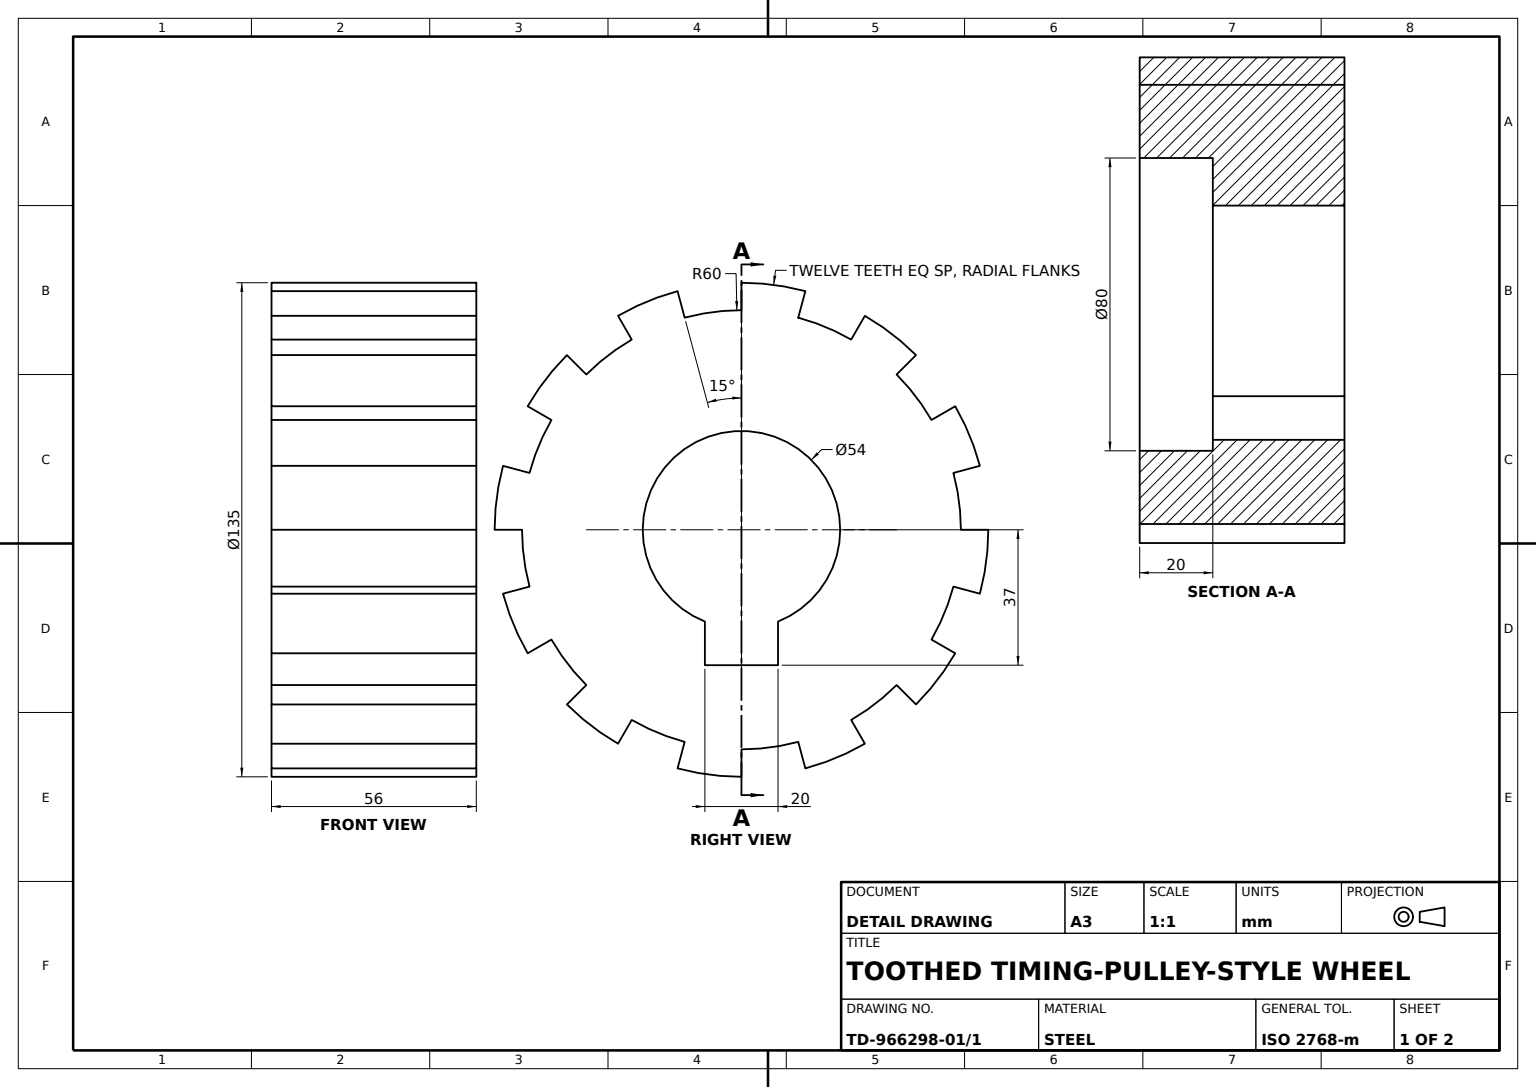
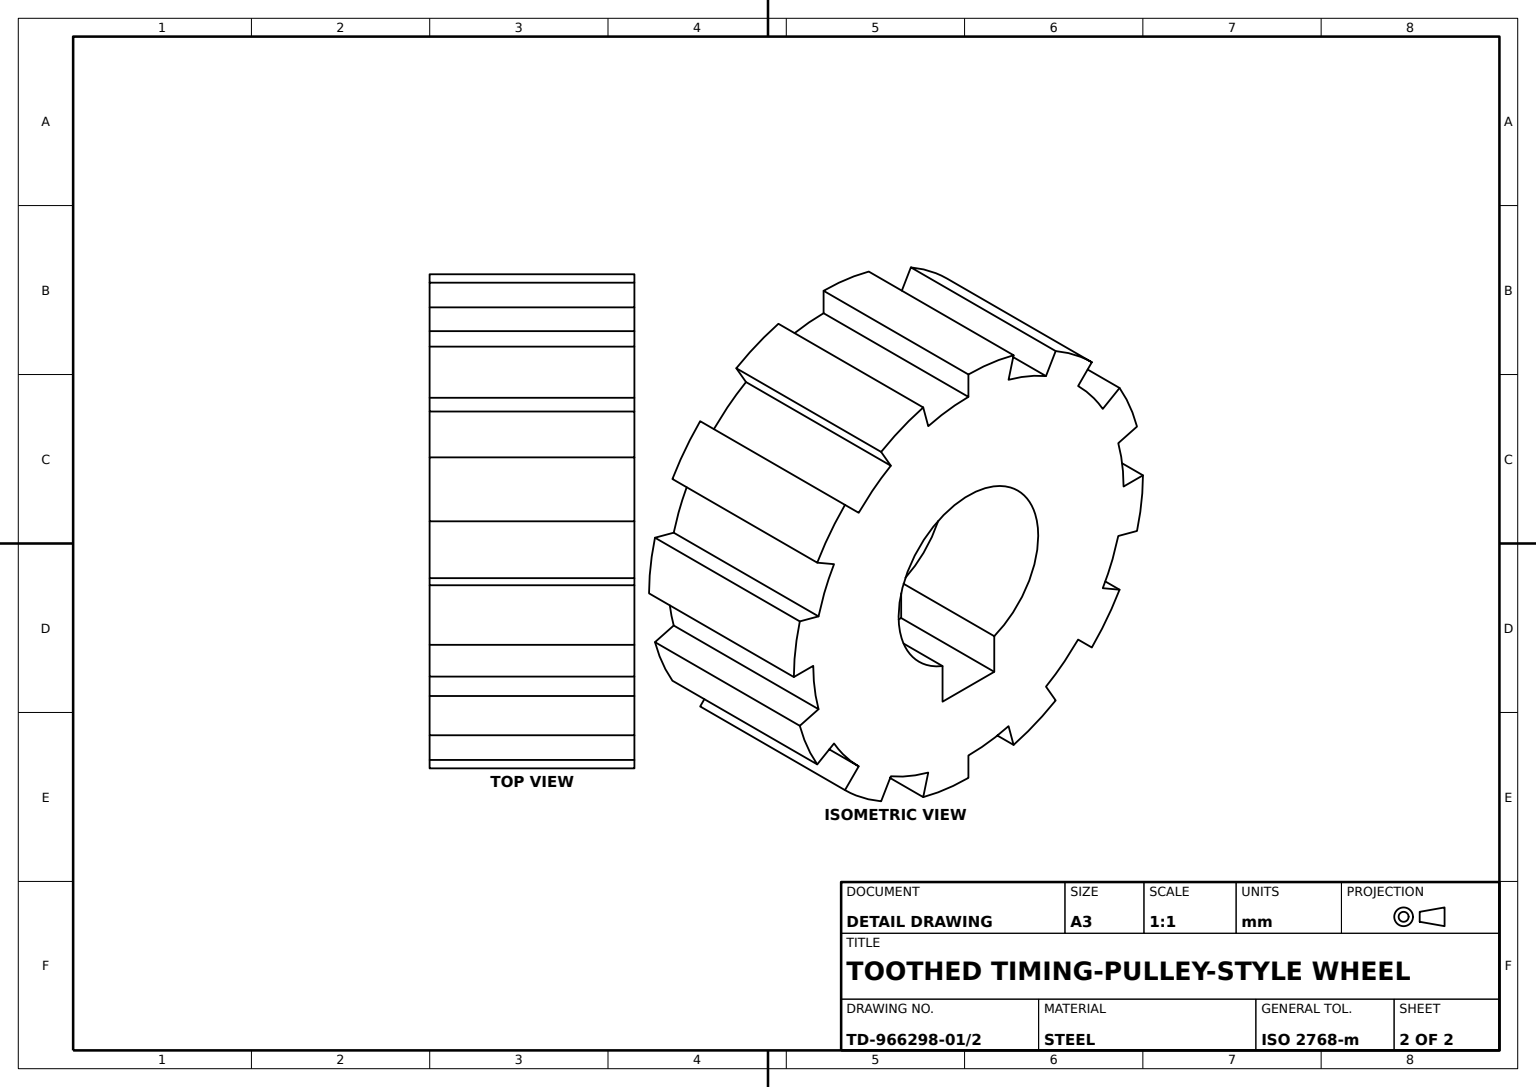
solid
v1 (10,-37,-56)
v2 (10,-37,-20)
e1 v1 v2 LINE
v3 (10,-25.079872,-20)
e2 v2 v3 LINE
v4 (10,-25.079872,-56)
e3 v4 v3 LINE
e4 v1 v4 LINE
face PLANE(AX(P(10,-37,-56),D(1,0,0),D(0,0,-1))) rev [e1 e2 -e3 -e4]
v5 (-47.729708,-47.729708,-56)
v6 (-47.729708,-47.729708,0)
e5 v5 v6 LINE
v7 (-42.426407,-42.426407,-56)
e6 v7 v5 LINE
v8 (-42.426407,-42.426407,0)
e7 v7 v8 LINE
e8 v8 v6 LINE
face PLANE(AX(P(0,0,-56),D(-0.707106781,0.707106781,0),D(-0.707106781,-0.707106781,0))) rev [-e5 -e6 e7 e8]
v9 (57.95555,-15.529143,0)
v10 (60,0,0)
e9 v9 v10 CIRCLE(AX(P(0,0,0),D(0,0,1),D(1,0,0)),60)
v11 (57.95555,-15.529143,-56)
e10 v11 v9 LINE
v12 (60,0,-56)
e11 v11 v12 CIRCLE(AX(P(0,0,-56),D(0,0,1),D(1,0,0)),60)
e12 v12 v10 LINE
face CYL(AX(P(0,0,-56),D(0,0,1),D(1,0,0)),60) [-e9 -e10 e11 e12]
v13 (65.199993,-17.470286,-56)
v14 (65.199993,-17.470286,0)
e13 v13 v14 LINE
e14 v11 v13 LINE
e15 v9 v14 LINE
face PLANE(AX(P(0,0,-56),D(-0.258819045,-0.965925826,0),D(0.965925826,-0.258819045,0))) rev [-e13 -e14 e10 e15]
v15 (-57.95555,15.529143,-56)
v16 (-57.95555,15.529143,0)
e16 v15 v16 LINE
v17 (-60,0,-56)
e17 v15 v17 CIRCLE(AX(P(0,0,-56),D(0,0,1),D(1,0,0)),60)
v18 (-60,0,0)
e18 v17 v18 LINE
e19 v16 v18 CIRCLE(AX(P(0,0,0),D(0,0,1),D(1,0,0)),60)
face CYL(AX(P(0,0,-56),D(0,0,1),D(1,0,0)),60) [-e16 e17 e18 -e19]
v19 (17.470286,65.199993,-56)
v20 (17.470286,65.199993,0)
e20 v19 v20 LINE
v21 (15.529143,57.95555,-56)
e21 v21 v19 LINE
v22 (15.529143,57.95555,0)
e22 v21 v22 LINE
e23 v22 v20 LINE
face PLANE(AX(P(0,0,-56),D(0.965925826,-0.258819045,0),D(0.258819045,0.965925826,0))) rev [-e20 -e21 e22 e23]
v23 (58.456715,-33.75,0)
e24 v23 v14 CIRCLE(AX(P(0,0,0),D(0,0,1),D(1,0,0)),67.5)
v24 (58.456715,-33.75,-56)
e25 v24 v23 LINE
e26 v24 v13 CIRCLE(AX(P(0,0,-56),D(0,0,1),D(1,0,0)),67.5)
face CYL(AX(P(0,0,-56),D(0,0,1),D(1,0,0)),67.5) [-e24 -e25 e26 e13]
v25 (42.426407,-42.426407,-56)
v26 (47.729708,-47.729708,-56)
e27 v25 v26 LINE
v27 (42.426407,-42.426407,0)
e28 v25 v27 LINE
v28 (47.729708,-47.729708,0)
e29 v27 v28 LINE
e30 v26 v28 LINE
face PLANE(AX(P(0,0,-56),D(-0.707106781,-0.707106781,0),D(0.707106781,-0.707106781,0))) rev [-e27 e28 e29 -e30]
v29 (67.5,0,-56)
v30 (67.5,0,0)
e31 v29 v30 LINE
e32 v10 v30 LINE
e33 v12 v29 LINE
face PLANE(AX(P(0,0,-56),D(0,-1,0),D(1,0,0))) [e31 -e32 -e12 e33]
v31 (40,0,-20)
v32 (40,0,0)
e34 v31 v32 LINE
v33 (-40,0,-20)
e35 v33 v31 CIRCLE(AX(P(0,0,-20),D(0,0,1),D(1,0,0)),40)
v34 (-40,0,0)
e36 v33 v34 LINE
e37 v34 v32 CIRCLE(AX(P(0,0,0),D(0,0,1),D(1,0,0)),40)
face CYL(AX(P(0,0,-20),D(0,0,1),D(1,0,0)),40) rev [-e34 -e35 e36 e37]
v35 (-33.75,-58.456715,-56)
v36 (-17.470286,-65.199993,-56)
e38 v35 v36 CIRCLE(AX(P(0,0,-56),D(0,0,1),D(1,0,0)),67.5)
v37 (-17.470286,-65.199993,0)
e39 v36 v37 LINE
v38 (-33.75,-58.456715,0)
e40 v38 v37 CIRCLE(AX(P(0,0,0),D(0,0,1),D(1,0,0)),67.5)
e41 v35 v38 LINE
face CYL(AX(P(0,0,-56),D(0,0,1),D(1,0,0)),67.5) [e38 e39 -e40 -e41]
v39 (0,-67.5,0)
v40 (17.470286,-65.199993,0)
e42 v39 v40 CIRCLE(AX(P(0,0,0),D(0,0,1),D(1,0,0)),67.5)
v41 (0,-67.5,-56)
e43 v41 v39 LINE
v42 (17.470286,-65.199993,-56)
e44 v41 v42 CIRCLE(AX(P(0,0,-56),D(0,0,1),D(1,0,0)),67.5)
e45 v42 v40 LINE
face CYL(AX(P(0,0,-56),D(0,0,1),D(1,0,0)),67.5) [-e42 -e43 e44 e45]
v43 (0,-60,-56)
v44 (0,-60,0)
e46 v43 v44 LINE
v45 (-15.529143,-57.95555,0)
e47 v45 v44 CIRCLE(AX(P(0,0,0),D(0,0,1),D(1,0,0)),60)
v46 (-15.529143,-57.95555,-56)
e48 v46 v45 LINE
e49 v46 v43 CIRCLE(AX(P(0,0,-56),D(0,0,1),D(1,0,0)),60)
face CYL(AX(P(0,0,-56),D(0,0,1),D(1,0,0)),60) [e46 -e47 -e48 e49]
e50 v44 v39 LINE
e51 v43 v41 LINE
face PLANE(AX(P(0,0,-56),D(-1,0,0),D(0,-1,0))) [-e50 -e46 e51 e43]
v47 (-58.456715,33.75,-56)
v48 (-58.456715,33.75,0)
e52 v47 v48 LINE
v49 (-65.199993,17.470286,-56)
e53 v47 v49 CIRCLE(AX(P(0,0,-56),D(0,0,1),D(1,0,0)),67.5)
v50 (-65.199993,17.470286,0)
e54 v49 v50 LINE
e55 v48 v50 CIRCLE(AX(P(0,0,0),D(0,0,1),D(1,0,0)),67.5)
face CYL(AX(P(0,0,-56),D(0,0,1),D(1,0,0)),67.5) [-e52 e53 e54 -e55]
v51 (-30,-51.961524,-56)
e56 v51 v35 LINE
v52 (-30,-51.961524,0)
e57 v52 v38 LINE
e58 v51 v52 LINE
face PLANE(AX(P(0,0,-56),D(-0.866025404,0.5,0),D(-0.5,-0.866025404,0))) [e56 e41 -e57 -e58]
e59 v16 v50 LINE
e60 v15 v49 LINE
face PLANE(AX(P(0,0,-56),D(0.258819045,0.965925826,0),D(-0.965925826,0.258819045,0))) rev [e59 -e54 -e60 e16]
v53 (-57.95555,-15.529143,-56)
v54 (-57.95555,-15.529143,0)
e61 v53 v54 LINE
v55 (-51.961524,-30,-56)
e62 v53 v55 CIRCLE(AX(P(0,0,-56),D(0,0,1),D(1,0,0)),60)
v56 (-51.961524,-30,0)
e63 v55 v56 LINE
e64 v54 v56 CIRCLE(AX(P(0,0,0),D(0,0,1),D(1,0,0)),60)
face CYL(AX(P(0,0,-56),D(0,0,1),D(1,0,0)),60) [-e61 e62 e63 -e64]
v57 (-67.5,0,-56)
v58 (-65.199993,-17.470286,-56)
e65 v57 v58 CIRCLE(AX(P(0,0,-56),D(0,0,1),D(1,0,0)),67.5)
v59 (-65.199993,-17.470286,0)
e66 v58 v59 LINE
v60 (-67.5,0,0)
e67 v60 v59 CIRCLE(AX(P(0,0,0),D(0,0,1),D(1,0,0)),67.5)
e68 v57 v60 LINE
face CYL(AX(P(0,0,-56),D(0,0,1),D(1,0,0)),67.5) [e65 e66 -e67 -e68]
v61 (-33.75,58.456715,-56)
v62 (-33.75,58.456715,0)
e69 v61 v62 LINE
v63 (-30,51.961524,0)
e70 v63 v62 LINE
v64 (-30,51.961524,-56)
e71 v64 v63 LINE
e72 v64 v61 LINE
face PLANE(AX(P(0,0,-56),D(0.866025404,0.5,0),D(-0.5,0.866025404,0))) [e69 -e70 -e71 e72]
e73 v31 v33 CIRCLE(AX(P(0,0,-20),D(0,0,1),D(1,0,0)),40)
v65 (27,0,-20)
v66 (-27,0,-20)
e74 v65 v66 CIRCLE(AX(P(0,0,-20),D(0,0,1),D(1,0,0)),27)
e75 v3 v65 CIRCLE(AX(P(0,0,-20),D(0,0,1),D(1,0,0)),27)
v67 (-10,-37,-20)
e76 v67 v2 LINE
v68 (-10,-25.079872,-20)
e77 v68 v67 LINE
e78 v66 v68 CIRCLE(AX(P(0,0,-20),D(0,0,1),D(1,0,0)),27)
face PLANE(AX(P(0,0,-20),D(0,0,1),D(1,0,0))) [e35 e73] [-e74 -e75 -e2 -e76 -e77 -e78]
v69 (-15.529143,57.95555,0)
v70 (-17.470286,65.199993,0)
e79 v69 v70 LINE
v71 (-17.470286,65.199993,-56)
e80 v71 v70 LINE
v72 (-15.529143,57.95555,-56)
e81 v72 v71 LINE
e82 v72 v69 LINE
face PLANE(AX(P(0,0,-56),D(0.965925826,0.258819045,0),D(-0.258819045,0.965925826,0))) rev [e79 -e80 -e81 e82]
v73 (65.199993,17.470286,-56)
e83 v29 v73 CIRCLE(AX(P(0,0,-56),D(0,0,1),D(1,0,0)),67.5)
v74 (65.199993,17.470286,0)
e84 v73 v74 LINE
e85 v30 v74 CIRCLE(AX(P(0,0,0),D(0,0,1),D(1,0,0)),67.5)
face CYL(AX(P(0,0,-56),D(0,0,1),D(1,0,0)),67.5) [e83 e84 -e85 -e31]
v75 (30,-51.961524,-56)
v76 (30,-51.961524,0)
e86 v75 v76 LINE
v77 (15.529143,-57.95555,0)
e87 v77 v76 CIRCLE(AX(P(0,0,0),D(0,0,1),D(1,0,0)),60)
v78 (15.529143,-57.95555,-56)
e88 v78 v77 LINE
e89 v78 v75 CIRCLE(AX(P(0,0,-56),D(0,0,1),D(1,0,0)),60)
face CYL(AX(P(0,0,-56),D(0,0,1),D(1,0,0)),60) [e86 -e87 -e88 e89]
v79 (33.75,-58.456715,-56)
e90 v79 v26 CIRCLE(AX(P(0,0,-56),D(0,0,1),D(1,0,0)),67.5)
v80 (33.75,-58.456715,0)
e91 v80 v28 CIRCLE(AX(P(0,0,0),D(0,0,1),D(1,0,0)),67.5)
e92 v79 v80 LINE
face CYL(AX(P(0,0,-56),D(0,0,1),D(1,0,0)),67.5) [e90 e30 -e91 -e92]
v81 (33.75,58.456715,0)
e93 v81 v20 CIRCLE(AX(P(0,0,0),D(0,0,1),D(1,0,0)),67.5)
v82 (33.75,58.456715,-56)
e94 v82 v81 LINE
e95 v82 v19 CIRCLE(AX(P(0,0,-56),D(0,0,1),D(1,0,0)),67.5)
face CYL(AX(P(0,0,-56),D(0,0,1),D(1,0,0)),67.5) [e20 -e93 -e94 e95]
v83 (-58.456715,-33.75,-56)
v84 (-58.456715,-33.75,0)
e96 v83 v84 LINE
e97 v83 v5 CIRCLE(AX(P(0,0,-56),D(0,0,1),D(1,0,0)),67.5)
e98 v84 v6 CIRCLE(AX(P(0,0,0),D(0,0,1),D(1,0,0)),67.5)
face CYL(AX(P(0,0,-56),D(0,0,1),D(1,0,0)),67.5) [-e96 e97 e5 -e98]
v85 (51.961524,30,-56)
v86 (51.961524,30,0)
e99 v85 v86 LINE
v87 (57.95555,15.529143,0)
e100 v87 v86 CIRCLE(AX(P(0,0,0),D(0,0,1),D(1,0,0)),60)
v88 (57.95555,15.529143,-56)
e101 v88 v87 LINE
e102 v88 v85 CIRCLE(AX(P(0,0,-56),D(0,0,1),D(1,0,0)),60)
face CYL(AX(P(0,0,-56),D(0,0,1),D(1,0,0)),60) [e99 -e100 -e101 e102]
v89 (58.456715,33.75,-56)
v90 (58.456715,33.75,0)
e103 v89 v90 LINE
e104 v86 v90 LINE
e105 v85 v89 LINE
face PLANE(AX(P(0,0,-56),D(0.5,-0.866025404,0),D(0.866025404,0.5,0))) [e103 -e104 -e99 e105]
e106 v56 v84 LINE
e107 v55 v83 LINE
face PLANE(AX(P(0,0,-56),D(-0.5,0.866025404,0),D(-0.866025404,-0.5,0))) [-e106 -e63 e107 e96]
v91 (-27,0,-56)
v92 (-10,-25.079872,-56)
e108 v91 v92 CIRCLE(AX(P(0,0,-56),D(0,0,1),D(1,0,0)),27)
e109 v91 v66 LINE
e110 v92 v68 LINE
face CYL(AX(P(0,0,-56),D(0,0,1),D(1,0,0)),27) rev [-e108 e109 e78 -e110]
v93 (-51.961524,30,0)
e111 v93 v48 LINE
v94 (-51.961524,30,-56)
e112 v94 v93 LINE
e113 v94 v47 LINE
face PLANE(AX(P(0,0,-56),D(0.5,0.866025404,0),D(-0.866025404,0.5,0))) [-e111 -e112 e113 e52]
e114 v77 v40 LINE
e115 v78 v42 LINE
face PLANE(AX(P(0,0,-56),D(-0.965925826,-0.258819045,0),D(0.258819045,-0.965925826,0))) rev [e114 -e45 -e115 e88]
e116 v54 v59 LINE
e117 v53 v58 LINE
face PLANE(AX(P(0,0,-56),D(-0.258819045,0.965925826,0),D(-0.965925826,-0.258819045,0))) rev [e61 e116 -e66 -e117]
v95 (27,0,-56)
e118 v95 v65 LINE
e119 v4 v95 CIRCLE(AX(P(0,0,-56),D(0,0,1),D(1,0,0)),27)
face CYL(AX(P(0,0,-56),D(0,0,1),D(1,0,0)),27) rev [e3 e75 -e118 -e119]
v96 (-42.426407,42.426407,0)
e120 v96 v93 CIRCLE(AX(P(0,0,0),D(0,0,1),D(1,0,0)),60)
v97 (-42.426407,42.426407,-56)
e121 v97 v96 LINE
e122 v97 v94 CIRCLE(AX(P(0,0,-56),D(0,0,1),D(1,0,0)),60)
face CYL(AX(P(0,0,-56),D(0,0,1),D(1,0,0)),60) [-e120 -e121 e122 e112]
v98 (30,51.961524,-56)
v99 (30,51.961524,0)
e123 v98 v99 LINE
e124 v98 v82 LINE
e125 v99 v81 LINE
face PLANE(AX(P(0,0,-56),D(0.866025404,-0.5,0),D(0.5,0.866025404,0))) [-e123 e124 e94 -e125]
e126 v72 v64 CIRCLE(AX(P(0,0,-56),D(0,0,1),D(1,0,0)),60)
e127 v69 v63 CIRCLE(AX(P(0,0,0),D(0,0,1),D(1,0,0)),60)
face CYL(AX(P(0,0,-56),D(0,0,1),D(1,0,0)),60) [e126 e71 -e127 -e82]
v100 (51.961524,-30,-56)
e128 v100 v24 LINE
v101 (51.961524,-30,0)
e129 v101 v23 LINE
e130 v100 v101 LINE
face PLANE(AX(P(0,0,-56),D(-0.5,-0.866025404,0),D(0.866025404,-0.5,0))) [e128 e25 -e129 -e130]
e131 v95 v91 CIRCLE(AX(P(0,0,-56),D(0,0,1),D(1,0,0)),27)
face CYL(AX(P(0,0,-56),D(0,0,1),D(1,0,0)),27) rev [-e109 -e131 e118 e74]
e132 v32 v34 CIRCLE(AX(P(0,0,0),D(0,0,1),D(1,0,0)),40)
e133 v8 v52 CIRCLE(AX(P(0,0,0),D(0,0,1),D(1,0,0)),60)
e134 v45 v37 LINE
e135 v76 v80 LINE
e136 v27 v101 CIRCLE(AX(P(0,0,0),D(0,0,1),D(1,0,0)),60)
e137 v87 v74 LINE
v102 (47.729708,47.729708,0)
e138 v90 v102 CIRCLE(AX(P(0,0,0),D(0,0,1),D(1,0,0)),67.5)
v103 (42.426407,42.426407,0)
e139 v103 v102 LINE
e140 v103 v99 CIRCLE(AX(P(0,0,0),D(0,0,1),D(1,0,0)),60)
v104 (0,60,0)
e141 v22 v104 CIRCLE(AX(P(0,0,0),D(0,0,1),D(1,0,0)),60)
v105 (0,67.5,0)
e142 v104 v105 LINE
e143 v105 v70 CIRCLE(AX(P(0,0,0),D(0,0,1),D(1,0,0)),67.5)
v106 (-47.729708,47.729708,0)
e144 v62 v106 CIRCLE(AX(P(0,0,0),D(0,0,1),D(1,0,0)),67.5)
e145 v96 v106 LINE
e146 v18 v60 LINE
face PLANE(AX(P(0,0,0),D(0,0,1),D(1,0,0))) [-e132 -e37] [e133 e57 e40 -e134 e47 e50 e42 -e114 e87 e135 e91 -e29 e136 e129 e24 -e15 e9 e32 e85 -e137 e100 e104 e138 -e139 e140 e125 e93 -e23 e141 e142 e143 -e79 e127 e70 e144 -e145 e120 e111 e55 -e59 e19 e146 e67 -e116 e64 e106 e98 -e8]
e147 v46 v36 LINE
face PLANE(AX(P(0,0,-56),D(-0.965925826,0.258819045,0),D(-0.258819045,-0.965925826,0))) rev [-e147 e48 e134 -e39]
face CYL(AX(P(0,0,-20),D(0,0,1),D(1,0,0)),40) rev [-e73 e34 e132 -e36]
e148 v75 v79 LINE
face PLANE(AX(P(0,0,-56),D(-0.866025404,-0.5,0),D(0.5,-0.866025404,0))) [e92 -e135 -e86 e148]
v107 (0,67.5,-56)
e149 v107 v105 LINE
e150 v107 v71 CIRCLE(AX(P(0,0,-56),D(0,0,1),D(1,0,0)),67.5)
face CYL(AX(P(0,0,-56),D(0,0,1),D(1,0,0)),67.5) [e80 -e143 -e149 e150]
e151 v25 v100 CIRCLE(AX(P(0,0,-56),D(0,0,1),D(1,0,0)),60)
face CYL(AX(P(0,0,-56),D(0,0,1),D(1,0,0)),60) [-e136 -e28 e151 e130]
v108 (47.729708,47.729708,-56)
e152 v89 v108 CIRCLE(AX(P(0,0,-56),D(0,0,1),D(1,0,0)),67.5)
e153 v108 v102 LINE
face CYL(AX(P(0,0,-56),D(0,0,1),D(1,0,0)),67.5) [e152 e153 -e138 -e103]
v109 (-10,-37,-56)
e154 v109 v67 LINE
e155 v109 v1 LINE
face PLANE(AX(P(0,-37,-56),D(0,-1,0),D(0,0,-1))) rev [e154 e76 -e1 -e155]
e156 v7 v51 CIRCLE(AX(P(0,0,-56),D(0,0,1),D(1,0,0)),60)
face CYL(AX(P(0,0,-56),D(0,0,1),D(1,0,0)),60) [e58 -e133 -e7 e156]
v110 (0,60,-56)
e157 v110 v107 LINE
e158 v110 v104 LINE
face PLANE(AX(P(0,0,-56),D(1,0,0),D(0,0,-1))) [e157 e149 -e142 -e158]
e159 v92 v109 LINE
face PLANE(AX(P(-10,-37,-56),D(-1,0,0),D(0,0,1))) rev [-e159 e110 e77 -e154]
e160 v17 v57 LINE
face PLANE(AX(P(0,0,-56),D(0,1,0),D(-1,0,0))) [e160 e68 -e146 -e18]
v111 (42.426407,42.426407,-56)
e161 v111 v103 LINE
e162 v111 v98 CIRCLE(AX(P(0,0,-56),D(0,0,1),D(1,0,0)),60)
face CYL(AX(P(0,0,-56),D(0,0,1),D(1,0,0)),60) [e123 -e140 -e161 e162]
e163 v21 v110 CIRCLE(AX(P(0,0,-56),D(0,0,1),D(1,0,0)),60)
e164 v111 v108 LINE
e165 v88 v73 LINE
v112 (-47.729708,47.729708,-56)
e166 v97 v112 LINE
e167 v61 v112 CIRCLE(AX(P(0,0,-56),D(0,0,1),D(1,0,0)),67.5)
face PLANE(AX(P(0,0,-56),D(0,0,1),D(1,0,0))) rev [e81 -e150 -e157 -e163 e21 -e95 -e124 -e162 e164 -e152 -e105 -e102 e165 -e83 -e33 -e11 e14 -e26 -e128 -e151 e27 -e90 -e148 -e89 e115 -e44 -e51 -e49 e147 -e38 -e56 -e156 e6 -e97 -e107 -e62 e117 -e65 -e160 -e17 e60 -e53 -e113 -e122 e166 -e167 -e72 -e126] [e159 e155 e4 e119 e131 e108]
e168 v112 v106 LINE
face PLANE(AX(P(0,0,-56),D(0.707106781,0.707106781,0),D(-0.707106781,0.707106781,0))) rev [-e166 e121 e145 -e168]
face PLANE(AX(P(0,0,-56),D(0.707106781,-0.707106781,0),D(0.707106781,0.707106781,0))) rev [-e164 e161 e139 -e153]
face CYL(AX(P(0,0,-56),D(0,0,1),D(1,0,0)),60) [-e22 e163 e158 -e141]
face PLANE(AX(P(0,0,-56),D(0.258819045,-0.965925826,0),D(0.965925826,0.258819045,0))) rev [-e165 e101 e137 -e84]
face CYL(AX(P(0,0,-56),D(0,0,1),D(1,0,0)),67.5) [e168 -e144 -e69 e167]
